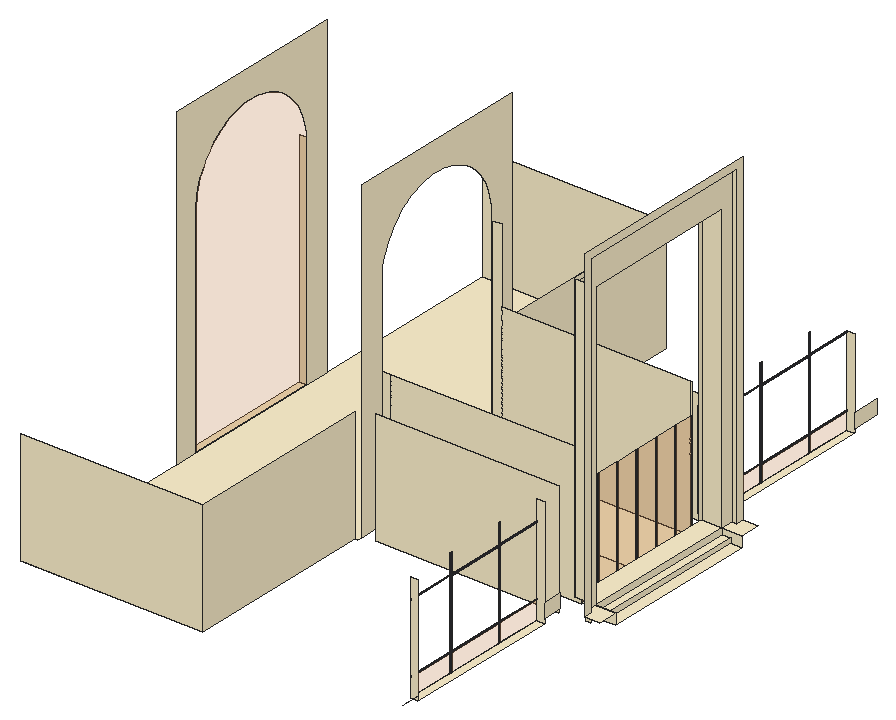
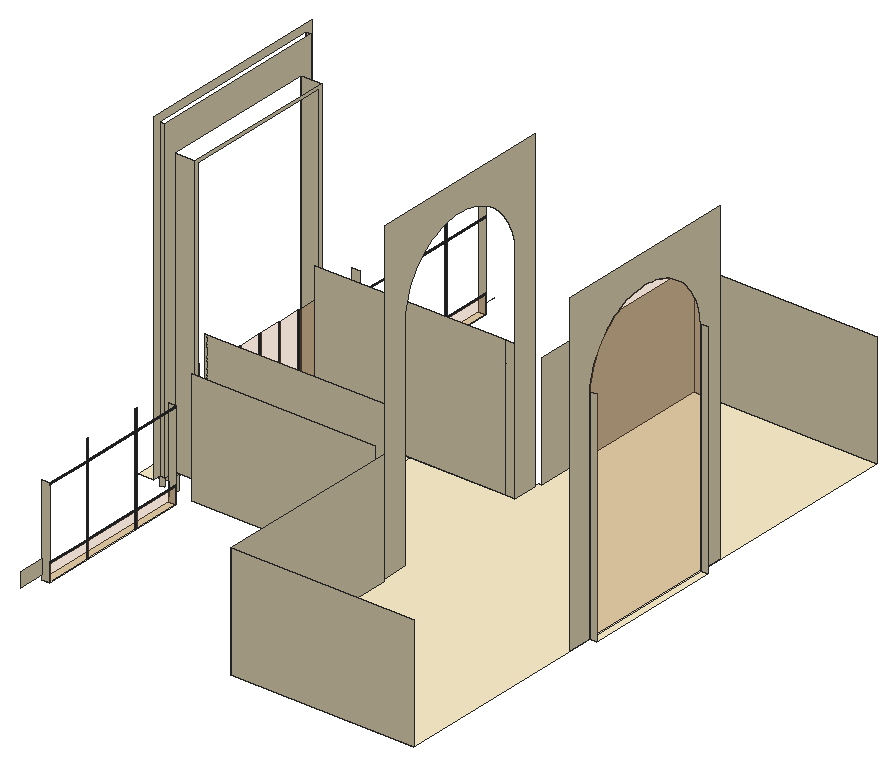
# SketchUp Ruby script. Lengths in inches.
U = 1.inch
M = Sketchup.active_model
def pt(a) = Geom::Point3d.new(a.map { |v| v * U })
def face(e, loops, mat)
  f = e.add_face(loops[0].map { |a| pt(a) })
  loops[1..].each { |l| e.add_face(l.map { |a| pt(a) }).erase! }
  f.material = f.back_material = mat if mat
  f
end
# faces: each face lists its corners as indices into pts; further lists are holes
def faces(e, pts, list, mat = nil) = list.each { |f| face(e, (f[0].is_a?(Array) ? f : [f]).map { |l| l.map { |i| pts[i] } }, mat) }
# xy, xz, yz: faces in a plane at the given z, y or x. An outline is a flat list of corners, or four numbers for a rectangle; further outlines are holes
def ring(l) = l.size == 4 ? [[l[0], l[1]], [l[2], l[1]], [l[2], l[3]], [l[0], l[3]]] : l.each_slice(2).to_a
def flat(e, list, mat, &to3) = list.each { |f| face(e, (f[0].is_a?(Array) ? f : [f]).map { |l| ring(l).map { |u, v| to3.(u, v) } }, mat) }
def xy(e, z, list, mat = nil) = flat(e, list, mat) { |x, y| [x, y, z] }
def xz(e, y, list, mat = nil) = flat(e, list, mat) { |x, z| [x, y, z] }
def yz(e, x, list, mat = nil) = flat(e, list, mat) { |y, z| [x, y, z] }
def lines(e, pts, list) = list.each { |a, b| e.add_line(pt(pts[a]), pt(pts[b])) }
# prism: a flat outline (further loops are holes) pulled along v
def prism(e, loops, v, mat = nil)
  f = face(e, loops, mat); d = Geom::Vector3d.new(v.map { |x| x * U })
  f.pushpull(f.normal.samedirection?(d) ? d.length : -d.length)
end
def box(e, o, s, mat = nil) = prism(e, [[o, [o[0] + s[0], o[1], o[2]], [o[0] + s[0], o[1] + s[1], o[2]], [o[0], o[1] + s[1], o[2]]]], [0, 0, s[2]], mat)
def at(x, y, z, deg = 0) = Geom::Transformation.translation(pt([x, y, z])) * Geom::Transformation.rotation(ORIGIN, Z_AXIS, deg.degrees)
def axes(o, x, y, z) = Geom::Transformation.new([*x, 0, *y, 0, *z, 0, *pt(o).to_a, 1])
def part(name) = M.definitions.add(name)
# library, detail: a bought-in or finely detailed component or shape, given as its bounding box
def library(name, o, s) = part(name).tap { |d| box(d.entities, o, s) }
def detail(e, o, s) = box(e.add_group.entities, o, s)
def put(e, d, t, mat = nil) = e.add_instance(d, t).tap { |i| i.material = mat if mat }
def group(e, t, mat = nil) = e.add_group.tap { |g| g.transformation = t; g.material = mat if mat }.entities
root = M.entities
M.materials.add("D01_Frost_White").color = [255, 242, 206]
M.materials.add("Glass_Safety_01").color = [244, 153, 81]
M.materials["Glass_Safety_01"].alpha = 0.25
M.materials.add("ThomThom - Buttons1").color = [48, 49, 53]
M.materials.add("ThomThom - Buttons2").color = [40, 40, 43]
xy(root,5.91,[[526,282,540.12,474]],"D01_Frost_White")
xy(root,6,[[21,27,243,27,243,258,246,258,246,294,373.5,294,373.5,342.01,373.02,342,370.76,342.1,368.52,342.35,366.29,342.73,364.09,343.25,361.92,343.91,359.81,344.71,357.74,345.63,355.74,346.69,353.81,347.86,351.96,349.16,350.1875,350.57,348.51,352.09,346.93,353.71,345.46,355.42,344.1,357.23,342.85,359.11,341.73,361.08,340.73,363.1,339.86,365.19,339.12,367.33,338.52,369.51,338.05,371.72,337.73,373.96,337.54,376.22,337.5,378.48,337.6,380.74,337.85,382.98,338.23,385.21,338.75,387.41,339.41,389.58,340.21,391.69,341.13,393.76,342.19,395.76,343.36,397.69,344.66,399.54,346.07,401.3125,347.59,402.99,349.21,404.57,350.92,406.04,352.73,407.4,354.61,408.65,356.58,409.77,358.6,410.77,360.69,411.64,362.83,412.38,365.01,412.98,367.22,413.45,369.46,413.77,371.72,413.96,373.5,413.99,373.5,462,246,462,246,498,243,498,243,729,21,729],[12,294,21,462],[373.5,294,489,294,489,378,409.49,378,409.5,377.52,409.4,375.26,409.15,373.02,408.77,370.79,408.25,368.59,407.59,366.42,406.79,364.31,405.87,362.24,404.81,360.24,403.64,358.31,402.34,356.46,400.93,354.6875,399.41,353.01,397.79,351.43,396.08,349.96,394.27,348.6,392.39,347.35,390.42,346.23,388.4,345.23,386.31,344.36,384.17,343.62,381.99,343.02,379.78,342.55,377.54,342.23,375.28,342.04,373.5,342.01],[409.49,378,489,378,489,462,373.5,462,373.5,413.99,373.98,414,376.24,413.9,378.48,413.65,380.71,413.27,382.91,412.75,385.08,412.09,387.19,411.29,389.26,410.37,391.26,409.31,393.19,408.14,395.04,406.84,396.8125,405.43,398.49,403.91,400.07,402.29,401.54,400.58,402.9,398.77,404.15,396.89,405.27,394.92,406.27,392.9,407.14,390.81,407.88,388.67,408.48,386.49,408.95,384.28,409.27,382.04,409.46,379.78]],"D01_Frost_White")
xy(root,11.82,[[516,282,526,474]],"D01_Frost_White")
xy(root,12,[[483,42,492,234],[483,513,492,705]],"D01_Frost_White")
xy(root,18,[[[373.02,342,373.5,342.01,375.28,342.04,377.54,342.23,379.78,342.55,381.99,343.02,384.17,343.62,386.31,344.36,388.4,345.23,390.42,346.23,392.39,347.35,394.27,348.6,396.08,349.96,397.79,351.43,399.41,353.01,400.93,354.6875,402.34,356.46,403.64,358.31,404.81,360.24,405.87,362.24,406.79,364.31,407.59,366.42,408.25,368.59,408.77,370.79,409.15,373.02,409.4,375.26,409.5,377.52,409.49,378,409.46,379.78,409.27,382.04,408.95,384.28,408.48,386.49,407.88,388.67,407.14,390.81,406.27,392.9,405.27,394.92,404.15,396.89,402.9,398.77,401.54,400.58,400.07,402.29,398.49,403.91,396.8125,405.43,395.04,406.84,393.19,408.14,391.26,409.31,389.26,410.37,387.19,411.29,385.08,412.09,382.91,412.75,380.71,413.27,378.48,413.65,376.24,413.9,373.98,414,373.5,413.99,371.72,413.96,369.46,413.77,367.22,413.45,365.01,412.98,362.83,412.38,360.69,411.64,358.6,410.77,356.58,409.77,354.61,408.65,352.73,407.4,350.92,406.04,349.21,404.57,347.59,402.99,346.07,401.3125,344.66,399.54,343.36,397.69,342.19,395.76,341.13,393.76,340.21,391.69,339.41,389.58,338.75,387.41,338.23,385.21,337.85,382.98,337.6,380.74,337.5,378.48,337.54,376.22,337.73,373.96,338.05,371.72,338.52,369.51,339.12,367.33,339.86,365.19,340.73,363.1,341.73,361.08,342.85,359.11,344.1,357.23,345.46,355.42,346.93,353.71,348.51,352.09,350.1875,350.57,351.96,349.16,353.81,347.86,355.74,346.69,357.74,345.63,359.81,344.71,361.92,343.91,364.09,343.25,366.29,342.73,368.52,342.35,370.76,342.1],[373.18,354.01,371.68,354.08,370.18,354.24,368.69,354.49,367.23,354.84,365.78,355.28,364.37,355.81,363,356.43,361.66,357.13,360.375,357.91,359.14,358.78,357.96,359.72,356.84,360.73,355.79,361.81,354.8125,362.95,353.9,364.15,353.07,365.41,352.32,366.72,351.66,368.07,351.08,369.46,350.58,370.89,350.18,372.34,349.875,373.82,349.66,375.31,349.54,376.8125,349.51,378.32,349.58,379.82,349.74,381.32,349.99,382.81,350.34,384.27,350.78,385.72,351.31,387.13,351.93,388.5,352.63,389.84,353.41,391.125,354.28,392.36,355.22,393.54,356.23,394.66,357.31,395.71,358.45,396.6875,359.65,397.6,360.91,398.43,362.22,399.18,363.57,399.84,364.96,400.42,366.39,400.92,367.84,401.32,369.32,401.625,370.81,401.84,372.3125,401.96,373.72,401.99,373.82,401.99,375.32,401.92,376.82,401.76,378.31,401.51,379.77,401.16,381.22,400.72,382.63,400.19,384,399.57,385.34,398.87,386.625,398.09,387.86,397.22,389.04,396.28,390.16,395.27,391.21,394.19,392.1875,393.05,393.1,391.85,393.93,390.59,394.68,389.28,395.34,387.93,395.92,386.54,396.42,385.11,396.82,383.66,397.125,382.18,397.34,380.69,397.46,379.1875,397.49,377.78,397.49,377.68,397.42,376.18,397.26,374.68,397.01,373.19,396.66,371.73,396.22,370.28,395.69,368.87,395.07,367.5,394.37,366.16,393.59,364.875,392.72,363.64,391.78,362.46,390.77,361.34,389.69,360.29,388.55,359.3125,387.35,358.4,386.09,357.57,384.78,356.82,383.43,356.16,382.04,355.58,380.61,355.08,379.16,354.68,377.68,354.375,376.19,354.16,374.6875,354.04,373.28,354.01]]],"D01_Frost_White")
xy(root,19.19,[[522,258,540.12,258,540.12,282,516,282,516,267,522,267],[491,282,516,474],[516,474,540.12,474,540.12,498,522,498,522,489,516,489]],"D01_Frost_White")
xy(root,30,[[[373.18,354.01,373.28,354.01,374.6875,354.04,376.19,354.16,377.68,354.375,379.16,354.68,380.61,355.08,382.04,355.58,383.43,356.16,384.78,356.82,386.09,357.57,387.35,358.4,388.55,359.3125,389.69,360.29,390.77,361.34,391.78,362.46,392.72,363.64,393.59,364.875,394.37,366.16,395.07,367.5,395.69,368.87,396.22,370.28,396.66,371.73,397.01,373.19,397.26,374.68,397.42,376.18,397.49,377.68,397.49,377.78,397.46,379.1875,397.34,380.69,397.125,382.18,396.82,383.66,396.42,385.11,395.92,386.54,395.34,387.93,394.68,389.28,393.93,390.59,393.1,391.85,392.1875,393.05,391.21,394.19,390.16,395.27,389.04,396.28,387.86,397.22,386.625,398.09,385.34,398.87,384,399.57,382.63,400.19,381.22,400.72,379.77,401.16,378.31,401.51,376.82,401.76,375.32,401.92,373.82,401.99,373.72,401.99,372.3125,401.96,370.81,401.84,369.32,401.625,367.84,401.32,366.39,400.92,364.96,400.42,363.57,399.84,362.22,399.18,360.91,398.43,359.65,397.6,358.45,396.6875,357.31,395.71,356.23,394.66,355.22,393.54,354.28,392.36,353.41,391.125,352.63,389.84,351.93,388.5,351.31,387.13,350.78,385.72,350.34,384.27,349.99,382.81,349.74,381.32,349.58,379.82,349.51,378.32,349.54,376.8125,349.66,375.31,349.875,373.82,350.18,372.34,350.58,370.89,351.08,369.46,351.66,368.07,352.32,366.72,353.07,365.41,353.9,364.15,354.8125,362.95,355.79,361.81,356.84,360.73,357.96,359.72,359.14,358.78,360.375,357.91,361.66,357.13,363,356.43,364.37,355.81,365.78,355.28,367.23,354.84,368.69,354.49,370.18,354.24,371.68,354.08],[373.34,366.01,372.59,366.05,371.84,366.13,371.1,366.25,370.37,366.43,369.64,366.65,368.94,366.91,368.25,367.22,367.59,367.57,366.94,367.96,366.33,368.4,365.74,368.86,365.18,369.37,364.65,369.91,364.16,370.48,363.71,371.08,363.29,371.71,362.92,372.36,362.59,373.04,362.3,373.73,362.05,374.45,361.85,375.17,361.7,375.91,361.59,376.66,361.53,377.41,361.51,378.16,361.55,378.91,361.63,379.66,361.75,380.4,361.93,381.13,362.15,381.86,362.41,382.56,362.72,383.25,363.07,383.91,363.46,384.56,363.9,385.17,364.36,385.76,364.87,386.32,365.41,386.85,365.98,387.34,366.58,387.79,367.21,388.21,367.86,388.58,368.54,388.91,369.23,389.2,369.95,389.45,370.67,389.65,371.41,389.8,372.16,389.91,372.91,389.97,373.66,389.99,374.41,389.95,375.16,389.87,375.9,389.75,376.63,389.57,377.36,389.35,378.06,389.09,378.75,388.78,379.41,388.43,380.06,388.04,380.67,387.6,381.26,387.14,381.82,386.63,382.35,386.09,382.84,385.52,383.29,384.92,383.71,384.29,384.08,383.64,384.41,382.96,384.7,382.27,384.95,381.55,385.15,380.83,385.3,380.09,385.41,379.34,385.47,378.59,385.49,377.84,385.45,377.09,385.37,376.34,385.25,375.6,385.07,374.87,384.85,374.14,384.59,373.44,384.28,372.75,383.93,372.09,383.54,371.44,383.1,370.83,382.64,370.24,382.13,369.68,381.59,369.15,381.02,368.66,380.42,368.21,379.79,367.79,379.14,367.42,378.46,367.09,377.77,366.8,377.05,366.55,376.33,366.35,375.59,366.2,374.84,366.09,374.09,366.03]]],"D01_Frost_White")
xz(root,27,[[21,6,243,144]],"D01_Frost_White")
xz(root,42,[[483,12,492,144]],"D01_Frost_White")
xz(root,234,[[483,12,492,144]],"D01_Frost_White")
xz(root,267,[[261,6,483,144],[516,9,522,19.19],[516,19.19,522,405]],"D01_Frost_White")
xz(root,282,[[526,5.91,526,11.82,516,11.82,516,19.19,540.12,19.19,540.12,5.91],[491,19.19,516,366]],"D01_Frost_White")
xz(root,286,[[490,28,491,144]],"D01_Frost_White")
xz(root,294,[[12,6,21,275.43],[246,6,258,174],[258,6,489,174]],"D01_Frost_White")
xz(root,354.01,[[373.18,18,373.28,30]],"D01_Frost_White")
xz(root,401.99,[[373.72,18,373.82,30]],"D01_Frost_White")
xz(root,462,[[12,6,21,275.43],[246,6,258,264],[258,6,486,174],[486,6,489,174]],"D01_Frost_White")
xz(root,470,[[490,28,491,144]],"D01_Frost_White")
xz(root,474,[[526,5.91,540.12,5.91,540.12,19.19,516,19.19,516,11.82,526,11.82],[491,19.19,516,366]],"D01_Frost_White")
xz(root,489,[[261,6,483,144],[516,9,522,19.19],[516,19.19,522,405]],"D01_Frost_White")
xz(root,513,[[483,12,492,120]],"D01_Frost_White")
xz(root,705,[[483,12,492,120]],"D01_Frost_White")
xz(root,729,[[21,6,243,144]],"D01_Frost_White")
yz(root,21,[[264,6,294,6,294,275.43,294.49,280.53,295.37,285.98,296.61,291.37,298.2,296.65,300.13,301.83,302.4,306.86,304.99,311.74,307.89,316.43,311.1,320.93,314.59,325.2,318.36,329.24,322.39,333.02,326.65,336.53,331.13,339.75,335.82,342.67,340.6875,345.28,345.71,347.5625,350.88,349.51,356.16,351.12,361.54,352.375,366.99,353.28,372.48,353.82,378,354,383.52,353.82,389.01,353.28,394.46,352.375,399.84,351.12,405.12,349.51,410.29,347.5625,415.3125,345.28,420.18,342.67,424.87,339.75,429.35,336.53,433.61,333.02,437.64,329.24,441.41,325.2,444.9,320.93,448.11,316.43,451.01,311.74,453.6,306.86,455.87,301.83,457.8,296.65,459.39,291.37,460.63,285.98,461.51,280.53,462,275.43,462,6,492,6,492,390,264,390]],"D01_Frost_White")
yz(root,21,[[294,6,462,6,462,275.43,461.51,280.53,460.63,285.98,459.39,291.37,457.8,296.65,455.87,301.83,453.6,306.86,451.01,311.74,448.11,316.43,444.9,320.93,441.41,325.2,437.64,329.24,433.61,333.02,429.35,336.53,424.87,339.75,420.18,342.67,415.3125,345.28,410.29,347.5625,405.12,349.51,399.84,351.12,394.46,352.375,389.01,353.28,383.52,353.82,378,354,372.48,353.82,366.99,353.28,361.54,352.375,356.16,351.12,350.88,349.51,345.71,347.5625,340.6875,345.28,335.82,342.67,331.13,339.75,326.65,336.53,322.39,333.02,318.36,329.24,314.59,325.2,311.1,320.93,307.89,316.43,304.99,311.74,302.4,306.86,300.13,301.83,298.2,296.65,296.61,291.37,295.37,285.98,294.49,280.53,294,275.43]],"Glass_Safety_01")
yz(root,243,[[27,6,258,144],[498,6,729,144]],"D01_Frost_White")
yz(root,246,[[264,6,264,390,492,390,492,6,462,6,462,275.43,461.51,280.53,460.63,285.98,459.39,291.37,457.8,296.65,455.87,301.83,453.6,306.86,451.01,311.74,448.11,316.43,444.9,320.93,441.41,325.2,437.64,329.24,433.61,333.02,429.35,336.53,424.87,339.75,420.18,342.67,415.3125,345.28,410.29,347.5625,405.12,349.51,399.84,351.12,394.46,352.375,389.01,353.28,383.52,353.82,378,354,372.48,353.82,366.99,353.28,361.54,352.375,356.16,351.12,350.88,349.51,345.71,347.5625,340.6875,345.28,335.82,342.67,331.13,339.75,326.65,336.53,322.39,333.02,318.36,329.24,314.59,325.2,311.1,320.93,307.89,316.43,304.99,311.74,302.4,306.86,300.13,301.83,298.2,296.65,296.61,291.37,295.37,285.98,294.49,280.53,294,275.43,294,6]],"D01_Frost_White")
yz(root,397.49,[[377.68,18,377.78,30]],"D01_Frost_White")
yz(root,483,[[42,12,102,34],[104,12,176,34],[178,12,234,34],[513,12,573,32],[575,12,647,32],
  [649,12,705,32]],"Glass_Safety_01")
yz(root,483,[[[102,12,104,12,104,34,176,34,176,12,178,12,178,34,234,34,234,36,178,36,178,118,234,118,234,120,178,120,178,144,176,144,176,120,104,120,104,144,102,144,102,120,42,120,42,118,102,118,102,36,42,36,42,34,102,34],[104,36,176,118]],[[573,12,575,12,575,32,647,32,647,12,649,12,649,32,705,32,705,34,649,34,649,118,705,118,705,120,649,120,649,144,647,144,647,120,575,120,575,144,573,144,573,120,513,120,513,118,573,118,573,34,513,34,513,32,573,32],[575,34,647,118]]],"ThomThom - Buttons1")
yz(root,489,[[294,6,318,136.9],[438,6,462,136.9],[320,8,347.5,136.9],[348.5,8,377,136.9],[379,8,407.5,136.9],
  [408.5,8,436,136.9]],"Glass_Safety_01")
yz(root,489,[[377,8,379,136.9]],"ThomThom - Buttons1")
yz(root,489,[[318,6,438,6,438,136.9,436,136.9,436,8,320,8,320,136.9,318,136.9],[347.5,8,348.5,136.9],[407.5,8,408.5,136.9]],"ThomThom - Buttons2")
yz(root,491,[[282,19.19,286,19.19,286,362,470,362,470,19.19,474,19.19,474,366,282.07,366,282.07,342.73,282,342]],"D01_Frost_White")
yz(root,492,[[234,17.1875,258,34.38],[498,17.4,513,34.8],[705,17.4,738,34.8]],"D01_Frost_White")
yz(root,516,[[282,11.82,474,19.19],[267,19.19,282,19.19,282,366,474,366,474,19.19,489,19.19,489,405,267,405]],"D01_Frost_White")
yz(root,522,[[258,19.19,267,19.19,267,405,489,405,489,19.19,498,19.19,498,414,258,414]],"D01_Frost_White")
yz(root,526,[[282,5.91,474,11.82]],"D01_Frost_White")
p = [[370.76,342.1,6],[373.02,342,6],[373.02,342,18],[370.76,342.1,18],[373.5,342.01,6],[373.5,342.01,18],
  [375.28,342.04,6],[375.28,342.04,18],[377.54,342.23,6],[377.54,342.23,18],[368.52,342.35,6],[368.52,342.35,18],
  [379.78,342.55,6],[379.78,342.55,18],[366.29,342.73,6],[366.29,342.73,18],[381.99,343.02,6],[381.99,343.02,18],
  [364.09,343.25,6],[364.09,343.25,18],[384.17,343.62,6],[384.17,343.62,18],[361.92,343.91,6],[361.92,343.91,18],
  [386.31,344.36,6],[386.31,344.36,18],[359.81,344.71,6],[359.81,344.71,18],[388.4,345.23,6],[388.4,345.23,18],
  [357.74,345.63,6],[357.74,345.63,18],[390.42,346.23,6],[390.42,346.23,18],[355.74,346.69,6],[355.74,346.69,18],
  [392.39,347.35,6],[392.39,347.35,18],[353.81,347.86,6],[353.81,347.86,18],[394.27,348.6,6],[394.27,348.6,18],
  [351.96,349.16,6],[351.96,349.16,18],[396.08,349.96,6],[396.08,349.96,18],[350.1875,350.57,6],[350.1875,350.57,18],
  [397.79,351.43,6],[397.79,351.43,18],[348.51,352.09,6],[348.51,352.09,18],[399.41,353.01,6],[399.41,353.01,18],
  [346.93,353.71,6],[346.93,353.71,18],[400.93,354.6875,6],[400.93,354.6875,18],[345.46,355.42,6],[345.46,355.42,18],
  [402.34,356.46,6],[402.34,356.46,18],[344.1,357.23,6],[344.1,357.23,18],[403.64,358.31,6],[403.64,358.31,18],
  [342.85,359.11,6],[342.85,359.11,18],[404.81,360.24,6],[404.81,360.24,18],[341.73,361.08,6],[341.73,361.08,18],
  [405.87,362.24,6],[405.87,362.24,18],[340.73,363.1,6],[340.73,363.1,18],[406.79,364.31,6],[406.79,364.31,18],
  [339.86,365.19,6],[339.86,365.19,18],[407.59,366.42,6],[407.59,366.42,18],[339.12,367.33,6],[339.12,367.33,18],
  [408.25,368.59,6],[408.25,368.59,18],[338.52,369.51,6],[338.52,369.51,18],[408.77,370.79,6],[408.77,370.79,18],
  [338.05,371.72,6],[338.05,371.72,18],[409.15,373.02,6],[409.15,373.02,18],[337.73,373.96,6],[337.73,373.96,18],
  [409.4,375.26,6],[409.4,375.26,18],[337.54,376.22,6],[337.54,376.22,18],[409.5,377.52,6],[409.5,377.52,18],
  [337.5,378.48,6],[337.5,378.48,18],[409.49,378,6],[409.49,378,18],[409.46,379.78,6],[409.46,379.78,18],
  [337.6,380.74,6],[337.6,380.74,18],[409.27,382.04,6],[409.27,382.04,18],[337.85,382.98,6],[337.85,382.98,18],
  [408.95,384.28,6],[408.95,384.28,18],[338.23,385.21,6],[338.23,385.21,18],[408.48,386.49,6],[408.48,386.49,18],
  [338.75,387.41,6],[338.75,387.41,18],[407.88,388.67,6],[407.88,388.67,18],[339.41,389.58,6],[339.41,389.58,18],
  [407.14,390.81,6],[407.14,390.81,18],[340.21,391.69,6],[340.21,391.69,18],[406.27,392.9,6],[406.27,392.9,18],
  [341.13,393.76,6],[341.13,393.76,18],[405.27,394.92,6],[405.27,394.92,18],[342.19,395.76,6],[342.19,395.76,18],
  [404.15,396.89,6],[404.15,396.89,18],[343.36,397.69,6],[343.36,397.69,18],[402.9,398.77,6],[402.9,398.77,18],
  [344.66,399.54,6],[344.66,399.54,18],[401.54,400.58,6],[401.54,400.58,18],[346.07,401.3125,6],[346.07,401.3125,18],
  [400.07,402.29,6],[400.07,402.29,18],[347.59,402.99,6],[347.59,402.99,18],[398.49,403.91,6],[398.49,403.91,18],
  [349.21,404.57,6],[349.21,404.57,18],[396.8125,405.43,6],[396.8125,405.43,18],[350.92,406.04,6],[350.92,406.04,18],
  [395.04,406.84,6],[395.04,406.84,18],[352.73,407.4,6],[352.73,407.4,18],[393.19,408.14,6],[393.19,408.14,18],
  [354.61,408.65,6],[354.61,408.65,18],[391.26,409.31,6],[391.26,409.31,18],[356.58,409.77,6],[356.58,409.77,18],
  [389.26,410.37,6],[389.26,410.37,18],[358.6,410.77,6],[358.6,410.77,18],[387.19,411.29,6],[387.19,411.29,18],
  [360.69,411.64,6],[360.69,411.64,18],[385.08,412.09,6],[385.08,412.09,18],[362.83,412.38,6],[362.83,412.38,18],
  [382.91,412.75,6],[382.91,412.75,18],[365.01,412.98,6],[365.01,412.98,18],[380.71,413.27,6],[380.71,413.27,18],
  [367.22,413.45,6],[367.22,413.45,18],[378.48,413.65,6],[378.48,413.65,18],[369.46,413.77,6],[369.46,413.77,18],
  [376.24,413.9,6],[376.24,413.9,18],[371.72,413.96,6],[371.72,413.96,18],[373.98,414,6],[373.98,414,18],
  [373.5,413.99,6],[373.5,413.99,18],[371.68,354.08,18],[373.18,354.01,18],[373.18,354.01,30],[371.68,354.08,30],
  [373.28,354.01,18],[374.6875,354.04,18],[374.6875,354.04,30],[373.28,354.01,30],[376.19,354.16,18],[376.19,354.16,30],
  [370.18,354.24,18],[370.18,354.24,30],[368.69,354.49,18],[368.69,354.49,30],[377.68,354.375,18],[377.68,354.375,30],
  [379.16,354.68,18],[379.16,354.68,30],[367.23,354.84,18],[367.23,354.84,30],[380.61,355.08,18],[380.61,355.08,30],
  [365.78,355.28,18],[365.78,355.28,30],[382.04,355.58,18],[382.04,355.58,30],[364.37,355.81,18],[364.37,355.81,30],
  [383.43,356.16,18],[383.43,356.16,30],[363,356.43,18],[363,356.43,30],[384.78,356.82,18],[384.78,356.82,30],
  [361.66,357.13,18],[361.66,357.13,30],[386.09,357.57,18],[386.09,357.57,30],[360.375,357.91,18],[360.375,357.91,30],
  [387.35,358.4,18],[387.35,358.4,30],[359.14,358.78,18],[359.14,358.78,30],[388.55,359.3125,18],[388.55,359.3125,30],
  [357.96,359.72,18],[357.96,359.72,30],[389.69,360.29,18],[389.69,360.29,30],[356.84,360.73,18],[356.84,360.73,30],
  [390.77,361.34,18],[390.77,361.34,30],[355.79,361.81,18],[355.79,361.81,30],[391.78,362.46,18],[391.78,362.46,30],
  [354.8125,362.95,18],[354.8125,362.95,30],[392.72,363.64,18],[392.72,363.64,30],[353.9,364.15,18],[353.9,364.15,30],
  [393.59,364.875,18],[393.59,364.875,30],[353.07,365.41,18],[353.07,365.41,30],[394.37,366.16,18],[394.37,366.16,30],
  [352.32,366.72,18],[352.32,366.72,30],[395.07,367.5,18],[395.07,367.5,30],[351.66,368.07,18],[351.66,368.07,30],
  [395.69,368.87,18],[395.69,368.87,30],[351.08,369.46,18],[351.08,369.46,30],[396.22,370.28,18],[396.22,370.28,30],
  [350.58,370.89,18],[350.58,370.89,30],[396.66,371.73,18],[396.66,371.73,30],[350.18,372.34,18],[350.18,372.34,30],
  [397.01,373.19,18],[397.01,373.19,30],[349.875,373.82,18],[349.875,373.82,30],[397.26,374.68,18],[397.26,374.68,30],
  [349.66,375.31,18],[349.66,375.31,30],[397.42,376.18,18],[397.42,376.18,30],[349.54,376.8125,18],[349.54,376.8125,30],
  [397.49,377.68,18],[397.49,377.68,30],[349.51,378.32,18],[349.51,378.32,30],[397.49,377.78,18],[397.46,379.1875,18],
  [397.46,379.1875,30],[397.49,377.78,30],[349.58,379.82,18],[349.58,379.82,30],[397.34,380.69,18],[397.34,380.69,30],
  [349.74,381.32,18],[349.74,381.32,30],[397.125,382.18,18],[397.125,382.18,30],[349.99,382.81,18],[349.99,382.81,30],
  [396.82,383.66,18],[396.82,383.66,30],[350.34,384.27,18],[350.34,384.27,30],[396.42,385.11,18],[396.42,385.11,30],
  [350.78,385.72,18],[350.78,385.72,30],[395.92,386.54,18],[395.92,386.54,30],[351.31,387.13,18],[351.31,387.13,30],
  [395.34,387.93,18],[395.34,387.93,30],[351.93,388.5,18],[351.93,388.5,30],[394.68,389.28,18],[394.68,389.28,30],
  [352.63,389.84,18],[352.63,389.84,30],[393.93,390.59,18],[393.93,390.59,30],[353.41,391.125,18],[353.41,391.125,30],
  [393.1,391.85,18],[393.1,391.85,30],[354.28,392.36,18],[354.28,392.36,30],[392.1875,393.05,18],[392.1875,393.05,30],
  [355.22,393.54,18],[355.22,393.54,30],[391.21,394.19,18],[391.21,394.19,30],[356.23,394.66,18],[356.23,394.66,30],
  [390.16,395.27,18],[390.16,395.27,30],[357.31,395.71,18],[357.31,395.71,30],[389.04,396.28,18],[389.04,396.28,30],
  [358.45,396.6875,18],[358.45,396.6875,30],[387.86,397.22,18],[387.86,397.22,30],[359.65,397.6,18],[359.65,397.6,30],
  [386.625,398.09,18],[386.625,398.09,30],[360.91,398.43,18],[360.91,398.43,30],[385.34,398.87,18],[385.34,398.87,30],
  [362.22,399.18,18],[362.22,399.18,30],[384,399.57,18],[384,399.57,30],[363.57,399.84,18],[363.57,399.84,30],
  [382.63,400.19,18],[382.63,400.19,30],[364.96,400.42,18],[364.96,400.42,30],[381.22,400.72,18],[381.22,400.72,30],
  [366.39,400.92,18],[366.39,400.92,30],[379.77,401.16,18],[379.77,401.16,30],[367.84,401.32,18],[367.84,401.32,30],
  [378.31,401.51,18],[378.31,401.51,30],[369.32,401.625,18],[369.32,401.625,30],[376.82,401.76,18],[376.82,401.76,30],
  [370.81,401.84,18],[370.81,401.84,30],[372.3125,401.96,18],[372.3125,401.96,30],[375.32,401.92,18],[375.32,401.92,30],
  [373.82,401.99,18],[373.82,401.99,30],[373.72,401.99,18],[373.72,401.99,30],[371.84,366.13,30],[372.59,366.05,30],
  [372.59,366.05,42],[371.84,366.13,42],[373.34,366.01,30],[373.34,366.01,42],[374.09,366.03,30],[374.09,366.03,42],
  [374.84,366.09,30],[374.84,366.09,42],[371.1,366.25,30],[371.1,366.25,42],[375.59,366.2,30],[375.59,366.2,42],
  [376.33,366.35,30],[376.33,366.35,42],[370.37,366.43,30],[370.37,366.43,42],[369.64,366.65,30],[369.64,366.65,42],
  [377.05,366.55,30],[377.05,366.55,42],[368.94,366.91,30],[368.94,366.91,42],[377.77,366.8,30],[377.77,366.8,42],
  [378.46,367.09,30],[378.46,367.09,42],[368.25,367.22,30],[368.25,367.22,42],[379.14,367.42,30],[379.14,367.42,42],
  [367.59,367.57,30],[367.59,367.57,42],[379.79,367.79,30],[379.79,367.79,42],[366.94,367.96,30],[366.94,367.96,42],
  [380.42,368.21,30],[380.42,368.21,42],[366.33,368.4,30],[366.33,368.4,42],[381.02,368.66,30],[381.02,368.66,42],
  [365.74,368.86,30],[365.74,368.86,42],[381.59,369.15,30],[381.59,369.15,42],[365.18,369.37,30],[365.18,369.37,42],
  [382.13,369.68,30],[382.13,369.68,42],[364.65,369.91,30],[364.65,369.91,42],[382.64,370.24,30],[382.64,370.24,42],
  [364.16,370.48,30],[364.16,370.48,42],[383.1,370.83,30],[383.1,370.83,42],[363.71,371.08,30],[363.71,371.08,42],
  [383.54,371.44,30],[383.54,371.44,42],[363.29,371.71,30],[363.29,371.71,42],[383.93,372.09,30],[383.93,372.09,42],
  [362.92,372.36,30],[362.92,372.36,42],[384.28,372.75,30],[384.28,372.75,42],[362.59,373.04,30],[362.59,373.04,42],
  [384.59,373.44,30],[384.59,373.44,42],[362.3,373.73,30],[362.3,373.73,42],[384.85,374.14,30],[384.85,374.14,42],
  [362.05,374.45,30],[362.05,374.45,42],[385.07,374.87,30],[385.07,374.87,42],[361.85,375.17,30],[361.85,375.17,42],
  [385.25,375.6,30],[385.25,375.6,42],[361.7,375.91,30],[361.7,375.91,42],[385.37,376.34,30],[385.37,376.34,42],
  [361.59,376.66,30],[361.59,376.66,42],[385.45,377.09,30],[385.45,377.09,42],[361.53,377.41,30],[361.53,377.41,42],
  [385.49,377.84,30],[385.49,377.84,42],[361.51,378.16,30],[361.51,378.16,42],[385.47,378.59,30],[385.47,378.59,42],
  [361.55,378.91,30],[361.55,378.91,42],[385.41,379.34,30],[385.41,379.34,42],[361.63,379.66,30],[361.63,379.66,42],
  [385.3,380.09,30],[385.3,380.09,42],[361.75,380.4,30],[361.75,380.4,42],[385.15,380.83,30],[385.15,380.83,42],
  [361.93,381.13,30],[361.93,381.13,42],[384.95,381.55,30],[384.95,381.55,42],[362.15,381.86,30],[362.15,381.86,42],
  [384.7,382.27,30],[384.7,382.27,42],[362.41,382.56,30],[362.41,382.56,42],[384.41,382.96,30],[384.41,382.96,42],
  [362.72,383.25,30],[362.72,383.25,42],[384.08,383.64,30],[384.08,383.64,42],[363.07,383.91,30],[363.07,383.91,42],
  [383.71,384.29,30],[383.71,384.29,42],[363.46,384.56,30],[363.46,384.56,42],[383.29,384.92,30],[383.29,384.92,42],
  [363.9,385.17,30],[363.9,385.17,42],[382.84,385.52,30],[382.84,385.52,42],[364.36,385.76,30],[364.36,385.76,42],
  [382.35,386.09,30],[382.35,386.09,42],[364.87,386.32,30],[364.87,386.32,42],[381.82,386.63,30],[381.82,386.63,42],
  [365.41,386.85,30],[365.41,386.85,42],[381.26,387.14,30],[381.26,387.14,42],[365.98,387.34,30],[365.98,387.34,42],
  [380.67,387.6,30],[380.67,387.6,42],[366.58,387.79,30],[366.58,387.79,42],[380.06,388.04,30],[380.06,388.04,42],
  [367.21,388.21,30],[367.21,388.21,42],[379.41,388.43,30],[379.41,388.43,42],[367.86,388.58,30],[367.86,388.58,42],
  [378.75,388.78,30],[378.75,388.78,42],[368.54,388.91,30],[368.54,388.91,42],[378.06,389.09,30],[378.06,389.09,42],
  [369.23,389.2,30],[369.23,389.2,42],[377.36,389.35,30],[377.36,389.35,42],[369.95,389.45,30],[369.95,389.45,42],
  [370.67,389.65,30],[370.67,389.65,42],[376.63,389.57,30],[376.63,389.57,42],[371.41,389.8,30],[371.41,389.8,42],
  [375.9,389.75,30],[375.9,389.75,42],[375.16,389.87,30],[375.16,389.87,42],[372.16,389.91,30],[372.16,389.91,42],
  [372.91,389.97,30],[372.91,389.97,42],[374.41,389.95,30],[374.41,389.95,42],[373.66,389.99,30],[373.66,389.99,42],
  [492,18,17.26],[492,42,17.26],[483,489,6],[483,462,6]]
faces(root,p,[[0,1,2,3],[1,4,5,2],[4,6,7,5],[6,8,9,7],[10,0,3,11],[8,12,13,9],[14,10,11,15],[12,16,17,13],
  [18,14,15,19],[16,20,21,17],[22,18,19,23],[20,24,25,21],[26,22,23,27],[24,28,29,25],[30,26,27,31],[28,32,33,29],
  [34,30,31,35],[32,36,37,33],[38,34,35,39],[36,40,41,37],[42,38,39,43],[40,44,45,41],[46,42,43,47],[44,48,49,45],
  [50,46,47,51],[48,52,53,49],[54,50,51,55],[52,56,57,53],[58,54,55,59],[56,60,61,57],[62,58,59,63],[60,64,65,61],
  [66,62,63,67],[64,68,69,65],[70,66,67,71],[68,72,73,69],[74,70,71,75],[72,76,77,73],[78,74,75,79],[76,80,81,77],
  [82,78,79,83],[80,84,85,81],[86,82,83,87],[84,88,89,85],[90,86,87,91],[88,92,93,89],[94,90,91,95],[92,96,97,93],
  [98,94,95,99],[96,100,101,97],[102,98,99,103],[100,104,105,101],[104,106,107,105],[108,102,103,109],[106,110,111,107],[112,108,109,113],
  [110,114,115,111],[116,112,113,117],[114,118,119,115],[120,116,117,121],[118,122,123,119],[124,120,121,125],[122,126,127,123],[128,124,125,129],
  [126,130,131,127],[132,128,129,133],[130,134,135,131],[136,132,133,137],[134,138,139,135],[140,136,137,141],[138,142,143,139],[144,140,141,145],
  [142,146,147,143],[148,144,145,149],[146,150,151,147],[152,148,149,153],[150,154,155,151],[156,152,153,157],[154,158,159,155],[160,156,157,161],
  [158,162,163,159],[164,160,161,165],[162,166,167,163],[168,164,165,169],[166,170,171,167],[172,168,169,173],[170,174,175,171],[176,172,173,177],
  [174,178,179,175],[180,176,177,181],[178,182,183,179],[184,180,181,185],[182,186,187,183],[188,184,185,189],[186,190,191,187],[192,188,189,193],
  [190,194,195,191],[196,192,193,197],[194,198,199,195],[200,196,197,201],[198,202,203,199],[204,200,201,205],[202,204,205,203],[206,207,208,209],
  [210,211,212,213],[211,214,215,212],[216,206,209,217],[218,216,217,219],[214,220,221,215],[220,222,223,221],[224,218,219,225],[222,226,227,223],
  [228,224,225,229],[226,230,231,227],[232,228,229,233],[230,234,235,231],[236,232,233,237],[234,238,239,235],[240,236,237,241],[238,242,243,239],
  [244,240,241,245],[242,246,247,243],[248,244,245,249],[246,250,251,247],[252,248,249,253],[250,254,255,251],[256,252,253,257],[254,258,259,255],
  [260,256,257,261],[258,262,263,259],[264,260,261,265],[262,266,267,263],[268,264,265,269],[266,270,271,267],[272,268,269,273],[270,274,275,271],
  [276,272,273,277],[274,278,279,275],[280,276,277,281],[278,282,283,279],[284,280,281,285],[282,286,287,283],[288,284,285,289],[286,290,291,287],
  [292,288,289,293],[290,294,295,291],[296,292,293,297],[294,298,299,295],[300,296,297,301],[298,302,303,299],[304,300,301,305],[302,306,307,303],
  [308,304,305,309],[310,311,312,313],[314,308,309,315],[311,316,317,312],[318,314,315,319],[316,320,321,317],[322,318,319,323],[320,324,325,321],
  [326,322,323,327],[324,328,329,325],[330,326,327,331],[328,332,333,329],[334,330,331,335],[332,336,337,333],[338,334,335,339],[336,340,341,337],
  [342,338,339,343],[340,344,345,341],[346,342,343,347],[344,348,349,345],[350,346,347,351],[348,352,353,349],[354,350,351,355],[352,356,357,353],
  [358,354,355,359],[356,360,361,357],[362,358,359,363],[360,364,365,361],[366,362,363,367],[364,368,369,365],[370,366,367,371],[368,372,373,369],
  [374,370,371,375],[372,376,377,373],[378,374,375,379],[376,380,381,377],[382,378,379,383],[380,384,385,381],[386,382,383,387],[384,388,389,385],
  [390,386,387,391],[388,392,393,389],[394,390,391,395],[392,396,397,393],[398,394,395,399],[396,400,401,397],[402,398,399,403],[404,402,403,405],
  [400,406,407,401],[406,408,409,407],[410,404,405,411],[412,413,414,415],[413,416,417,414],[416,418,419,417],[418,420,421,419],[422,412,415,423],
  [420,424,425,421],[424,426,427,425],[428,422,423,429],[430,428,429,431],[426,432,433,427],[434,430,431,435],[432,436,437,433],[436,438,439,437],
  [440,434,435,441],[438,442,443,439],[444,440,441,445],[442,446,447,443],[448,444,445,449],[446,450,451,447],[452,448,449,453],[450,454,455,451],
  [456,452,453,457],[454,458,459,455],[460,456,457,461],[458,462,463,459],[464,460,461,465],[462,466,467,463],[468,464,465,469],[466,470,471,467],
  [472,468,469,473],[470,474,475,471],[476,472,473,477],[474,478,479,475],[480,476,477,481],[478,482,483,479],[484,480,481,485],[482,486,487,483],
  [488,484,485,489],[486,490,491,487],[492,488,489,493],[490,494,495,491],[496,492,493,497],[494,498,499,495],[500,496,497,501],[498,502,503,499],
  [504,500,501,505],[502,506,507,503],[508,504,505,509],[506,510,511,507],[512,508,509,513],[510,514,515,511],[516,512,513,517],[514,518,519,515],
  [520,516,517,521],[518,522,523,519],[524,520,521,525],[522,526,527,523],[528,524,525,529],[526,530,531,527],[532,528,529,533],[530,534,535,531],
  [536,532,533,537],[534,538,539,535],[540,536,537,541],[538,542,543,539],[544,540,541,545],[542,546,547,543],[548,544,545,549],[546,550,551,547],
  [552,548,549,553],[550,554,555,551],[556,552,553,557],[554,558,559,555],[560,556,557,561],[558,562,563,559],[564,560,561,565],[562,566,567,563],
  [568,564,565,569],[566,570,571,567],[572,568,569,573],[570,574,575,571],[576,572,573,577],[574,578,579,575],[580,576,577,581],[578,582,583,579],
  [584,580,581,585],[582,586,587,583],[588,584,585,589],[586,590,591,587],[592,588,589,593],[594,592,593,595],[590,596,597,591],[598,594,595,599],
  [596,600,601,597],[600,602,603,601],[604,598,599,605],[606,604,605,607],[602,608,609,603],[610,606,607,611],[608,610,611,609]],"D01_Frost_White")
lines(root,p,[[612,613],[614,615]])
